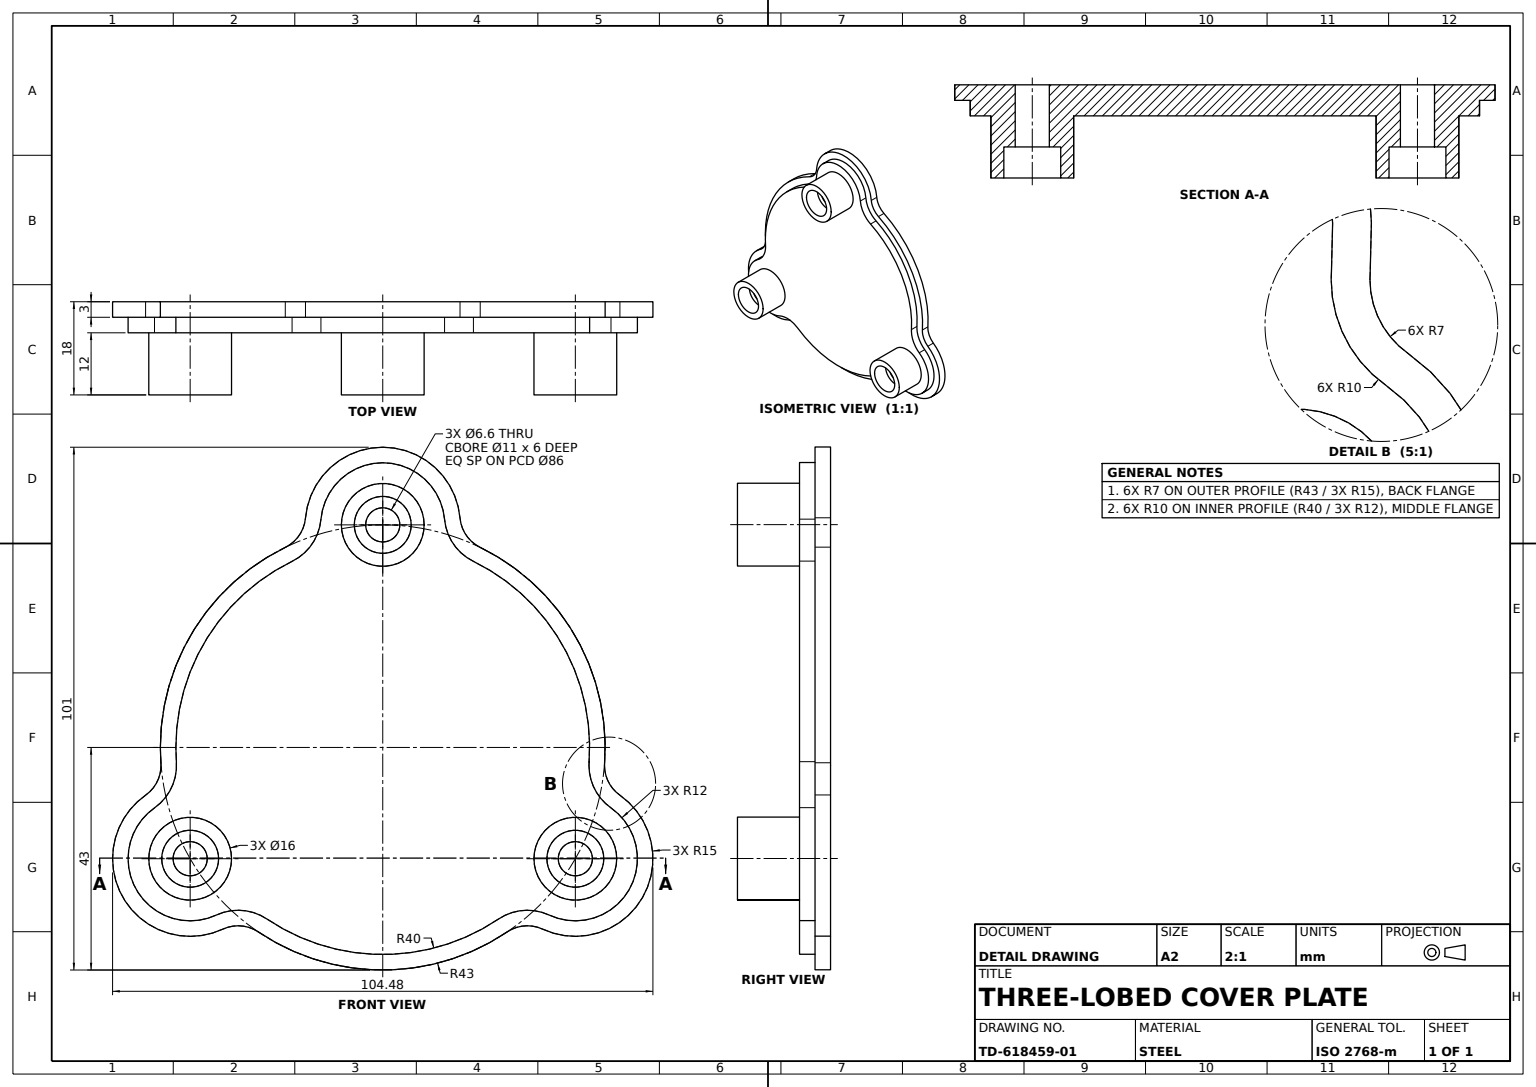
ISO-10303-21;
HEADER;
FILE_DESCRIPTION((''),'2;1');
FILE_NAME('','',(''),(''),'','','');
FILE_SCHEMA(('AUTOMOTIVE_DESIGN'));
ENDSEC;
DATA;
#1=APPLICATION_CONTEXT('');
#2=PRODUCT_CONTEXT('',#1,'mechanical');
#3=PRODUCT('','','',(#2));
#4=PRODUCT_DEFINITION_FORMATION('','',#3);
#5=PRODUCT_DEFINITION_CONTEXT('',#1,'design');
#6=PRODUCT_DEFINITION('','',#4,#5);
#7=PRODUCT_DEFINITION_SHAPE('','',#6);
#8=(LENGTH_UNIT()NAMED_UNIT(*)SI_UNIT(.MILLI.,.METRE.));
#9=(NAMED_UNIT(*)PLANE_ANGLE_UNIT()SI_UNIT($,.RADIAN.));
#10=(NAMED_UNIT(*)SI_UNIT($,.STERADIAN.)SOLID_ANGLE_UNIT());
#11=UNCERTAINTY_MEASURE_WITH_UNIT(LENGTH_MEASURE(1.E-05),#8,'distance_accuracy_value','');
#12=(GEOMETRIC_REPRESENTATION_CONTEXT(3)GLOBAL_UNCERTAINTY_ASSIGNED_CONTEXT((#11))GLOBAL_UNIT_ASSIGNED_CONTEXT((#8,#9,#10))REPRESENTATION_CONTEXT('',''));
#13=CARTESIAN_POINT('',(-31.739092,-21.5,12.));
#14=VERTEX_POINT('',#13);
#15=CARTESIAN_POINT('',(-31.739092,-21.5,18.));
#16=VERTEX_POINT('',#15);
#17=DIRECTION('',(0.,0.,1.));
#18=VECTOR('',#17,1000.);
#19=LINE('',#13,#18);
#20=EDGE_CURVE('',#14,#16,#19,.T.);
#21=ORIENTED_EDGE('',*,*,#20,.F.);
#22=CARTESIAN_POINT('',(-42.739092,-21.5,12.));
#23=VERTEX_POINT('',#22);
#24=CARTESIAN_POINT('',(-37.239092,-21.5,12.));
#25=DIRECTION('',(1.,0.,0.));
#26=AXIS2_PLACEMENT_3D('',#24,#17,#25);
#27=CIRCLE('',#26,5.5);
#28=EDGE_CURVE('',#23,#14,#27,.T.);
#29=ORIENTED_EDGE('',*,*,#28,.F.);
#30=CARTESIAN_POINT('',(-42.739092,-21.5,18.));
#31=VERTEX_POINT('',#30);
#32=LINE('',#22,#18);
#33=EDGE_CURVE('',#23,#31,#32,.T.);
#34=ORIENTED_EDGE('',*,*,#33,.T.);
#35=CARTESIAN_POINT('',(-37.239092,-21.5,18.));
#36=AXIS2_PLACEMENT_3D('',#35,#17,#25);
#37=CIRCLE('',#36,5.5);
#38=EDGE_CURVE('',#31,#16,#37,.T.);
#39=ORIENTED_EDGE('',*,*,#38,.T.);
#40=EDGE_LOOP('',(#21,#29,#34,#39));
#41=FACE_OUTER_BOUND('',#40,.T.);
#42=CYLINDRICAL_SURFACE('',#26,5.5);
#43=ADVANCED_FACE('',(#41),#42,.F.);
#44=CARTESIAN_POINT('',(-29.239092,-21.5,18.));
#45=VERTEX_POINT('',#44);
#46=CARTESIAN_POINT('',(-29.239092,-21.5,6.));
#47=VERTEX_POINT('',#46);
#48=DIRECTION('',(0.,0.,-1.));
#49=VECTOR('',#48,1000.);
#50=LINE('',#44,#49);
#51=EDGE_CURVE('',#45,#47,#50,.T.);
#52=ORIENTED_EDGE('',*,*,#51,.T.);
#53=CARTESIAN_POINT('',(-45.239092,-21.5,6.));
#54=VERTEX_POINT('',#53);
#55=CARTESIAN_POINT('',(-37.239092,-21.5,6.));
#56=AXIS2_PLACEMENT_3D('',#55,#17,#25);
#57=CIRCLE('',#56,8.);
#58=EDGE_CURVE('',#47,#54,#57,.T.);
#59=ORIENTED_EDGE('',*,*,#58,.T.);
#60=CARTESIAN_POINT('',(-45.239092,-21.5,18.));
#61=VERTEX_POINT('',#60);
#62=LINE('',#60,#49);
#63=EDGE_CURVE('',#61,#54,#62,.T.);
#64=ORIENTED_EDGE('',*,*,#63,.F.);
#65=CIRCLE('',#36,8.);
#66=EDGE_CURVE('',#45,#61,#65,.T.);
#67=ORIENTED_EDGE('',*,*,#66,.F.);
#68=EDGE_LOOP('',(#52,#59,#64,#67));
#69=FACE_OUTER_BOUND('',#68,.T.);
#70=DIRECTION('',(-1.,0.,0.));
#71=AXIS2_PLACEMENT_3D('',#35,#48,#70);
#72=CYLINDRICAL_SURFACE('',#71,8.);
#73=ADVANCED_FACE('',(#69),#72,.T.);
#74=CARTESIAN_POINT('',(-8.,43.,18.));
#75=VERTEX_POINT('',#74);
#76=CARTESIAN_POINT('',(8.,43.,18.));
#77=VERTEX_POINT('',#76);
#78=CARTESIAN_POINT('',(0.,43.,18.));
#79=AXIS2_PLACEMENT_3D('',#78,#17,#25);
#80=CIRCLE('',#79,8.);
#81=EDGE_CURVE('',#75,#77,#80,.T.);
#82=ORIENTED_EDGE('',*,*,#81,.F.);
#83=CARTESIAN_POINT('',(-8.,43.,6.));
#84=VERTEX_POINT('',#83);
#85=LINE('',#74,#49);
#86=EDGE_CURVE('',#75,#84,#85,.T.);
#87=ORIENTED_EDGE('',*,*,#86,.T.);
#88=CARTESIAN_POINT('',(8.,43.,6.));
#89=VERTEX_POINT('',#88);
#90=CARTESIAN_POINT('',(0.,43.,6.));
#91=AXIS2_PLACEMENT_3D('',#90,#17,#25);
#92=CIRCLE('',#91,8.);
#93=EDGE_CURVE('',#84,#89,#92,.T.);
#94=ORIENTED_EDGE('',*,*,#93,.T.);
#95=LINE('',#76,#49);
#96=EDGE_CURVE('',#77,#89,#95,.T.);
#97=ORIENTED_EDGE('',*,*,#96,.F.);
#98=EDGE_LOOP('',(#82,#87,#94,#97));
#99=FACE_OUTER_BOUND('',#98,.T.);
#100=AXIS2_PLACEMENT_3D('',#78,#48,#70);
#101=CYLINDRICAL_SURFACE('',#100,8.);
#102=ADVANCED_FACE('',(#99),#101,.T.);
#103=CARTESIAN_POINT('',(5.5,43.,18.));
#104=VERTEX_POINT('',#103);
#105=CARTESIAN_POINT('',(-5.5,43.,18.));
#106=VERTEX_POINT('',#105);
#107=CIRCLE('',#79,5.5);
#108=EDGE_CURVE('',#104,#106,#107,.T.);
#109=ORIENTED_EDGE('',*,*,#108,.T.);
#110=CARTESIAN_POINT('',(-5.5,43.,12.));
#111=VERTEX_POINT('',#110);
#112=LINE('',#110,#18);
#113=EDGE_CURVE('',#111,#106,#112,.T.);
#114=ORIENTED_EDGE('',*,*,#113,.F.);
#115=CARTESIAN_POINT('',(5.5,43.,12.));
#116=VERTEX_POINT('',#115);
#117=CARTESIAN_POINT('',(0.,43.,12.));
#118=AXIS2_PLACEMENT_3D('',#117,#17,#25);
#119=CIRCLE('',#118,5.5);
#120=EDGE_CURVE('',#116,#111,#119,.T.);
#121=ORIENTED_EDGE('',*,*,#120,.F.);
#122=LINE('',#115,#18);
#123=EDGE_CURVE('',#116,#104,#122,.T.);
#124=ORIENTED_EDGE('',*,*,#123,.T.);
#125=EDGE_LOOP('',(#109,#114,#121,#124));
#126=FACE_OUTER_BOUND('',#125,.T.);
#127=CYLINDRICAL_SURFACE('',#118,5.5);
#128=ADVANCED_FACE('',(#126),#127,.F.);
#129=CARTESIAN_POINT('',(-30.91498,-35.101676,3.));
#130=VERTEX_POINT('',#129);
#131=CARTESIAN_POINT('',(-24.048805,-35.646248,3.));
#132=VERTEX_POINT('',#131);
#133=CARTESIAN_POINT('',(-27.963727,-41.449125,3.));
#134=AXIS2_PLACEMENT_3D('',#133,#48,#70);
#135=CIRCLE('',#134,7.);
#136=EDGE_CURVE('',#130,#132,#135,.T.);
#137=ORIENTED_EDGE('',*,*,#136,.F.);
#138=CARTESIAN_POINT('',(-30.91498,-35.101676,0.));
#139=VERTEX_POINT('',#138);
#140=LINE('',#129,#49);
#141=EDGE_CURVE('',#130,#139,#140,.T.);
#142=ORIENTED_EDGE('',*,*,#141,.T.);
#143=CARTESIAN_POINT('',(-24.048805,-35.646248,0.));
#144=VERTEX_POINT('',#143);
#145=CARTESIAN_POINT('',(-27.963727,-41.449125,0.));
#146=AXIS2_PLACEMENT_3D('',#145,#48,#70);
#147=CIRCLE('',#146,7.);
#148=EDGE_CURVE('',#139,#144,#147,.T.);
#149=ORIENTED_EDGE('',*,*,#148,.T.);
#150=LINE('',#131,#49);
#151=EDGE_CURVE('',#132,#144,#150,.T.);
#152=ORIENTED_EDGE('',*,*,#151,.F.);
#153=EDGE_LOOP('',(#137,#142,#149,#152));
#154=FACE_OUTER_BOUND('',#153,.T.);
#155=CYLINDRICAL_SURFACE('',#134,7.);
#156=ADVANCED_FACE('',(#154),#155,.F.);
#157=CARTESIAN_POINT('',(39.877859,-3.492735,6.));
#158=VERTEX_POINT('',#157);
#159=CARTESIAN_POINT('',(39.877859,-3.492735,3.));
#160=VERTEX_POINT('',#159);
#161=LINE('',#157,#49);
#162=EDGE_CURVE('',#158,#160,#161,.T.);
#163=ORIENTED_EDGE('',*,*,#162,.F.);
#164=CARTESIAN_POINT('',(44.132965,-11.677856,6.));
#165=VERTEX_POINT('',#164);
#166=CARTESIAN_POINT('',(49.877859,-3.492735,6.));
#167=AXIS2_PLACEMENT_3D('',#166,#17,#25);
#168=CIRCLE('',#167,10.);
#169=EDGE_CURVE('',#158,#165,#168,.T.);
#170=ORIENTED_EDGE('',*,*,#169,.T.);
#171=CARTESIAN_POINT('',(44.132965,-11.677856,3.));
#172=VERTEX_POINT('',#171);
#173=LINE('',#164,#49);
#174=EDGE_CURVE('',#165,#172,#173,.T.);
#175=ORIENTED_EDGE('',*,*,#174,.T.);
#176=CARTESIAN_POINT('',(49.877859,-3.492735,3.));
#177=AXIS2_PLACEMENT_3D('',#176,#17,#25);
#178=CIRCLE('',#177,10.);
#179=EDGE_CURVE('',#160,#172,#178,.T.);
#180=ORIENTED_EDGE('',*,*,#179,.F.);
#181=EDGE_LOOP('',(#163,#170,#175,#180));
#182=FACE_OUTER_BOUND('',#181,.T.);
#183=AXIS2_PLACEMENT_3D('',#166,#48,#70);
#184=CYLINDRICAL_SURFACE('',#183,10.);
#185=ADVANCED_FACE('',(#182),#184,.F.);
#186=CARTESIAN_POINT('',(3.3,43.,0.));
#187=VERTEX_POINT('',#186);
#188=CARTESIAN_POINT('',(3.3,43.,12.));
#189=VERTEX_POINT('',#188);
#190=CARTESIAN_POINT('',(3.3,43.,-134.));
#191=LINE('',#190,#18);
#192=EDGE_CURVE('',#187,#189,#191,.T.);
#193=ORIENTED_EDGE('',*,*,#192,.F.);
#194=CARTESIAN_POINT('',(-3.3,43.,0.));
#195=VERTEX_POINT('',#194);
#196=CARTESIAN_POINT('',(0.,43.,0.));
#197=AXIS2_PLACEMENT_3D('',#196,#48,#70);
#198=CIRCLE('',#197,3.3);
#199=EDGE_CURVE('',#187,#195,#198,.T.);
#200=ORIENTED_EDGE('',*,*,#199,.T.);
#201=CARTESIAN_POINT('',(-3.3,43.,12.));
#202=VERTEX_POINT('',#201);
#203=CARTESIAN_POINT('',(-3.3,43.,-134.));
#204=LINE('',#203,#18);
#205=EDGE_CURVE('',#195,#202,#204,.T.);
#206=ORIENTED_EDGE('',*,*,#205,.T.);
#207=CIRCLE('',#118,3.3);
#208=EDGE_CURVE('',#202,#189,#207,.T.);
#209=ORIENTED_EDGE('',*,*,#208,.T.);
#210=EDGE_LOOP('',(#193,#200,#206,#209));
#211=FACE_OUTER_BOUND('',#210,.T.);
#212=CARTESIAN_POINT('',(0.,43.,-134.));
#213=AXIS2_PLACEMENT_3D('',#212,#17,#25);
#214=CYLINDRICAL_SURFACE('',#213,3.3);
#215=ADVANCED_FACE('',(#211),#214,.F.);
#216=CARTESIAN_POINT('',(45.239092,-21.5,18.));
#217=VERTEX_POINT('',#216);
#218=CARTESIAN_POINT('',(29.239092,-21.5,18.));
#219=VERTEX_POINT('',#218);
#220=CARTESIAN_POINT('',(37.239092,-21.5,18.));
#221=AXIS2_PLACEMENT_3D('',#220,#17,#25);
#222=CIRCLE('',#221,8.);
#223=EDGE_CURVE('',#217,#219,#222,.T.);
#224=ORIENTED_EDGE('',*,*,#223,.F.);
#225=CARTESIAN_POINT('',(45.239092,-21.5,6.));
#226=VERTEX_POINT('',#225);
#227=LINE('',#216,#49);
#228=EDGE_CURVE('',#217,#226,#227,.T.);
#229=ORIENTED_EDGE('',*,*,#228,.T.);
#230=CARTESIAN_POINT('',(29.239092,-21.5,6.));
#231=VERTEX_POINT('',#230);
#232=CARTESIAN_POINT('',(37.239092,-21.5,6.));
#233=AXIS2_PLACEMENT_3D('',#232,#17,#25);
#234=CIRCLE('',#233,8.);
#235=EDGE_CURVE('',#226,#231,#234,.T.);
#236=ORIENTED_EDGE('',*,*,#235,.T.);
#237=LINE('',#218,#49);
#238=EDGE_CURVE('',#219,#231,#237,.T.);
#239=ORIENTED_EDGE('',*,*,#238,.F.);
#240=EDGE_LOOP('',(#224,#229,#236,#239));
#241=FACE_OUTER_BOUND('',#240,.T.);
#242=AXIS2_PLACEMENT_3D('',#220,#48,#70);
#243=CYLINDRICAL_SURFACE('',#242,8.);
#244=ADVANCED_FACE('',(#241),#243,.T.);
#245=CARTESIAN_POINT('',(22.370982,-33.1593,6.));
#246=VERTEX_POINT('',#245);
#247=CARTESIAN_POINT('',(22.370982,-33.1593,3.));
#248=VERTEX_POINT('',#247);
#249=LINE('',#245,#49);
#250=EDGE_CURVE('',#246,#248,#249,.T.);
#251=ORIENTED_EDGE('',*,*,#250,.T.);
#252=CARTESIAN_POINT('',(32.179802,-32.381341,3.));
#253=VERTEX_POINT('',#252);
#254=CARTESIAN_POINT('',(27.963727,-41.449125,3.));
#255=AXIS2_PLACEMENT_3D('',#254,#17,#25);
#256=CIRCLE('',#255,10.);
#257=EDGE_CURVE('',#253,#248,#256,.T.);
#258=ORIENTED_EDGE('',*,*,#257,.F.);
#259=CARTESIAN_POINT('',(32.179802,-32.381341,6.));
#260=VERTEX_POINT('',#259);
#261=LINE('',#259,#49);
#262=EDGE_CURVE('',#260,#253,#261,.T.);
#263=ORIENTED_EDGE('',*,*,#262,.F.);
#264=CARTESIAN_POINT('',(27.963727,-41.449125,6.));
#265=AXIS2_PLACEMENT_3D('',#264,#17,#25);
#266=CIRCLE('',#265,10.);
#267=EDGE_CURVE('',#260,#246,#266,.T.);
#268=ORIENTED_EDGE('',*,*,#267,.T.);
#269=EDGE_LOOP('',(#251,#258,#263,#268));
#270=FACE_OUTER_BOUND('',#269,.T.);
#271=AXIS2_PLACEMENT_3D('',#264,#48,#70);
#272=CYLINDRICAL_SURFACE('',#271,10.);
#273=ADVANCED_FACE('',(#270),#272,.F.);
#274=CARTESIAN_POINT('',(-40.,0.,6.));
#275=VERTEX_POINT('',#274);
#276=CARTESIAN_POINT('',(-40.,0.,3.));
#277=VERTEX_POINT('',#276);
#278=LINE('',#274,#49);
#279=EDGE_CURVE('',#275,#277,#278,.T.);
#280=ORIENTED_EDGE('',*,*,#279,.F.);
#281=CARTESIAN_POINT('',(-17.531306,35.953488,6.));
#282=VERTEX_POINT('',#281);
#283=CARTESIAN_POINT('',(0.,0.,6.));
#284=AXIS2_PLACEMENT_3D('',#283,#17,#25);
#285=CIRCLE('',#284,40.);
#286=EDGE_CURVE('',#282,#275,#285,.T.);
#287=ORIENTED_EDGE('',*,*,#286,.F.);
#288=CARTESIAN_POINT('',(-17.531306,35.953488,3.));
#289=VERTEX_POINT('',#288);
#290=LINE('',#281,#49);
#291=EDGE_CURVE('',#282,#289,#290,.T.);
#292=ORIENTED_EDGE('',*,*,#291,.T.);
#293=CARTESIAN_POINT('',(0.,0.,3.));
#294=AXIS2_PLACEMENT_3D('',#293,#17,#25);
#295=CIRCLE('',#294,40.);
#296=EDGE_CURVE('',#289,#277,#295,.T.);
#297=ORIENTED_EDGE('',*,*,#296,.T.);
#298=EDGE_LOOP('',(#280,#287,#292,#297));
#299=FACE_OUTER_BOUND('',#298,.T.);
#300=AXIS2_PLACEMENT_3D('',#283,#48,#70);
#301=CYLINDRICAL_SURFACE('',#300,40.);
#302=ADVANCED_FACE('',(#299),#301,.T.);
#303=CARTESIAN_POINT('',(40.539092,-21.5,12.));
#304=VERTEX_POINT('',#303);
#305=CARTESIAN_POINT('',(33.939092,-21.5,12.));
#306=VERTEX_POINT('',#305);
#307=CARTESIAN_POINT('',(37.239092,-21.5,12.));
#308=AXIS2_PLACEMENT_3D('',#307,#17,#25);
#309=CIRCLE('',#308,3.3);
#310=EDGE_CURVE('',#304,#306,#309,.T.);
#311=ORIENTED_EDGE('',*,*,#310,.F.);
#312=EDGE_CURVE('',#306,#304,#309,.T.);
#313=ORIENTED_EDGE('',*,*,#312,.F.);
#314=EDGE_LOOP('',(#311,#313));
#315=FACE_BOUND('',#314,.T.);
#316=CARTESIAN_POINT('',(31.739092,-21.5,12.));
#317=VERTEX_POINT('',#316);
#318=CARTESIAN_POINT('',(42.739092,-21.5,12.));
#319=VERTEX_POINT('',#318);
#320=CIRCLE('',#308,5.5);
#321=EDGE_CURVE('',#317,#319,#320,.T.);
#322=ORIENTED_EDGE('',*,*,#321,.T.);
#323=EDGE_CURVE('',#319,#317,#320,.T.);
#324=ORIENTED_EDGE('',*,*,#323,.T.);
#325=EDGE_LOOP('',(#322,#324));
#326=FACE_OUTER_BOUND('',#325,.T.);
#327=PLANE('',#308);
#328=ADVANCED_FACE('',(#315,#326),#327,.T.);
#329=CARTESIAN_POINT('',(11.953163,44.059197,6.));
#330=VERTEX_POINT('',#329);
#331=CARTESIAN_POINT('',(-11.953163,44.059197,6.));
#332=VERTEX_POINT('',#331);
#333=CIRCLE('',#91,12.);
#334=EDGE_CURVE('',#330,#332,#333,.T.);
#335=ORIENTED_EDGE('',*,*,#334,.F.);
#336=CARTESIAN_POINT('',(11.953163,44.059197,3.));
#337=VERTEX_POINT('',#336);
#338=LINE('',#329,#49);
#339=EDGE_CURVE('',#330,#337,#338,.T.);
#340=ORIENTED_EDGE('',*,*,#339,.T.);
#341=CARTESIAN_POINT('',(-11.953163,44.059197,3.));
#342=VERTEX_POINT('',#341);
#343=CARTESIAN_POINT('',(0.,43.,3.));
#344=AXIS2_PLACEMENT_3D('',#343,#17,#25);
#345=CIRCLE('',#344,12.);
#346=EDGE_CURVE('',#337,#342,#345,.T.);
#347=ORIENTED_EDGE('',*,*,#346,.T.);
#348=LINE('',#331,#49);
#349=EDGE_CURVE('',#332,#342,#348,.T.);
#350=ORIENTED_EDGE('',*,*,#349,.F.);
#351=EDGE_LOOP('',(#335,#340,#347,#350));
#352=FACE_OUTER_BOUND('',#351,.T.);
#353=AXIS2_PLACEMENT_3D('',#90,#48,#70);
#354=CYLINDRICAL_SURFACE('',#353,12.);
#355=ADVANCED_FACE('',(#352),#354,.T.);
#356=CARTESIAN_POINT('',(-49.239092,-21.5,6.));
#357=VERTEX_POINT('',#356);
#358=CARTESIAN_POINT('',(-49.239092,-21.5,3.));
#359=VERTEX_POINT('',#358);
#360=LINE('',#356,#49);
#361=EDGE_CURVE('',#357,#359,#360,.T.);
#362=ORIENTED_EDGE('',*,*,#361,.T.);
#363=CARTESIAN_POINT('',(-32.179802,-32.381341,3.));
#364=VERTEX_POINT('',#363);
#365=CARTESIAN_POINT('',(-37.239092,-21.5,3.));
#366=AXIS2_PLACEMENT_3D('',#365,#17,#25);
#367=CIRCLE('',#366,12.);
#368=EDGE_CURVE('',#359,#364,#367,.T.);
#369=ORIENTED_EDGE('',*,*,#368,.T.);
#370=CARTESIAN_POINT('',(-32.179802,-32.381341,6.));
#371=VERTEX_POINT('',#370);
#372=LINE('',#370,#49);
#373=EDGE_CURVE('',#371,#364,#372,.T.);
#374=ORIENTED_EDGE('',*,*,#373,.F.);
#375=CIRCLE('',#56,12.);
#376=EDGE_CURVE('',#357,#371,#375,.T.);
#377=ORIENTED_EDGE('',*,*,#376,.F.);
#378=EDGE_LOOP('',(#362,#369,#374,#377));
#379=FACE_OUTER_BOUND('',#378,.T.);
#380=AXIS2_PLACEMENT_3D('',#55,#48,#70);
#381=CYLINDRICAL_SURFACE('',#380,12.);
#382=ADVANCED_FACE('',(#379),#381,.T.);
#383=CARTESIAN_POINT('',(-39.902287,-2.794188,6.));
#384=VERTEX_POINT('',#383);
#385=CARTESIAN_POINT('',(-39.902287,-2.794188,3.));
#386=VERTEX_POINT('',#385);
#387=LINE('',#383,#49);
#388=EDGE_CURVE('',#384,#386,#387,.T.);
#389=ORIENTED_EDGE('',*,*,#388,.T.);
#390=CARTESIAN_POINT('',(-44.132965,-11.677856,3.));
#391=VERTEX_POINT('',#390);
#392=CARTESIAN_POINT('',(-49.877859,-3.492735,3.));
#393=AXIS2_PLACEMENT_3D('',#392,#17,#25);
#394=CIRCLE('',#393,10.);
#395=EDGE_CURVE('',#391,#386,#394,.T.);
#396=ORIENTED_EDGE('',*,*,#395,.F.);
#397=CARTESIAN_POINT('',(-44.132965,-11.677856,6.));
#398=VERTEX_POINT('',#397);
#399=LINE('',#397,#49);
#400=EDGE_CURVE('',#398,#391,#399,.T.);
#401=ORIENTED_EDGE('',*,*,#400,.F.);
#402=CARTESIAN_POINT('',(-49.877859,-3.492735,6.));
#403=AXIS2_PLACEMENT_3D('',#402,#17,#25);
#404=CIRCLE('',#403,10.);
#405=EDGE_CURVE('',#398,#384,#404,.T.);
#406=ORIENTED_EDGE('',*,*,#405,.T.);
#407=EDGE_LOOP('',(#389,#396,#401,#406));
#408=FACE_OUTER_BOUND('',#407,.T.);
#409=AXIS2_PLACEMENT_3D('',#402,#48,#70);
#410=CYLINDRICAL_SURFACE('',#409,10.);
#411=ADVANCED_FACE('',(#408),#410,.F.);
#412=CARTESIAN_POINT('',(-42.894959,-3.003752,0.));
#413=VERTEX_POINT('',#412);
#414=CARTESIAN_POINT('',(-45.856433,-9.22232,0.));
#415=VERTEX_POINT('',#414);
#416=CARTESIAN_POINT('',(-49.877859,-3.492735,0.));
#417=AXIS2_PLACEMENT_3D('',#416,#48,#25);
#418=CIRCLE('',#417,7.);
#419=EDGE_CURVE('',#413,#415,#418,.T.);
#420=ORIENTED_EDGE('',*,*,#419,.T.);
#421=CARTESIAN_POINT('',(-45.856433,-9.22232,3.));
#422=VERTEX_POINT('',#421);
#423=LINE('',#421,#49);
#424=EDGE_CURVE('',#422,#415,#423,.T.);
#425=ORIENTED_EDGE('',*,*,#424,.F.);
#426=CARTESIAN_POINT('',(-42.894959,-3.003752,3.));
#427=VERTEX_POINT('',#426);
#428=AXIS2_PLACEMENT_3D('',#392,#48,#25);
#429=CIRCLE('',#428,7.);
#430=EDGE_CURVE('',#427,#422,#429,.T.);
#431=ORIENTED_EDGE('',*,*,#430,.F.);
#432=LINE('',#426,#49);
#433=EDGE_CURVE('',#427,#413,#432,.T.);
#434=ORIENTED_EDGE('',*,*,#433,.T.);
#435=EDGE_LOOP('',(#420,#425,#431,#434));
#436=FACE_OUTER_BOUND('',#435,.T.);
#437=AXIS2_PLACEMENT_3D('',#392,#48,#70);
#438=CYLINDRICAL_SURFACE('',#437,7.);
#439=ADVANCED_FACE('',(#436),#438,.F.);
#440=EDGE_CURVE('',#14,#23,#27,.T.);
#441=ORIENTED_EDGE('',*,*,#440,.T.);
#442=ORIENTED_EDGE('',*,*,#28,.T.);
#443=EDGE_LOOP('',(#441,#442));
#444=FACE_OUTER_BOUND('',#443,.T.);
#445=CARTESIAN_POINT('',(-40.539092,-21.5,12.));
#446=VERTEX_POINT('',#445);
#447=CARTESIAN_POINT('',(-33.939092,-21.5,12.));
#448=VERTEX_POINT('',#447);
#449=CIRCLE('',#26,3.3);
#450=EDGE_CURVE('',#446,#448,#449,.T.);
#451=ORIENTED_EDGE('',*,*,#450,.F.);
#452=EDGE_CURVE('',#448,#446,#449,.T.);
#453=ORIENTED_EDGE('',*,*,#452,.F.);
#454=EDGE_LOOP('',(#451,#453));
#455=FACE_BOUND('',#454,.T.);
#456=PLANE('',#26);
#457=ADVANCED_FACE('',(#444,#455),#456,.T.);
#458=CARTESIAN_POINT('',(-14.941454,44.323996,3.));
#459=VERTEX_POINT('',#458);
#460=CARTESIAN_POINT('',(-18.846153,38.65,3.));
#461=VERTEX_POINT('',#460);
#462=CARTESIAN_POINT('',(-21.914132,44.94186,3.));
#463=AXIS2_PLACEMENT_3D('',#462,#48,#70);
#464=CIRCLE('',#463,7.);
#465=EDGE_CURVE('',#459,#461,#464,.T.);
#466=ORIENTED_EDGE('',*,*,#465,.F.);
#467=CARTESIAN_POINT('',(-14.941454,44.323996,0.));
#468=VERTEX_POINT('',#467);
#469=LINE('',#458,#49);
#470=EDGE_CURVE('',#459,#468,#469,.T.);
#471=ORIENTED_EDGE('',*,*,#470,.T.);
#472=CARTESIAN_POINT('',(-18.846153,38.65,0.));
#473=VERTEX_POINT('',#472);
#474=CARTESIAN_POINT('',(-21.914132,44.94186,0.));
#475=AXIS2_PLACEMENT_3D('',#474,#48,#70);
#476=CIRCLE('',#475,7.);
#477=EDGE_CURVE('',#468,#473,#476,.T.);
#478=ORIENTED_EDGE('',*,*,#477,.T.);
#479=LINE('',#460,#49);
#480=EDGE_CURVE('',#461,#473,#479,.T.);
#481=ORIENTED_EDGE('',*,*,#480,.F.);
#482=EDGE_LOOP('',(#466,#471,#478,#481));
#483=FACE_OUTER_BOUND('',#482,.T.);
#484=CYLINDRICAL_SURFACE('',#463,7.);
#485=ADVANCED_FACE('',(#483),#484,.F.);
#486=CARTESIAN_POINT('',(-33.939092,-21.5,0.));
#487=VERTEX_POINT('',#486);
#488=CARTESIAN_POINT('',(-33.939092,-21.5,-134.));
#489=LINE('',#488,#18);
#490=EDGE_CURVE('',#487,#448,#489,.T.);
#491=ORIENTED_EDGE('',*,*,#490,.F.);
#492=CARTESIAN_POINT('',(-40.539092,-21.5,0.));
#493=VERTEX_POINT('',#492);
#494=CARTESIAN_POINT('',(-37.239092,-21.5,0.));
#495=AXIS2_PLACEMENT_3D('',#494,#48,#70);
#496=CIRCLE('',#495,3.3);
#497=EDGE_CURVE('',#487,#493,#496,.T.);
#498=ORIENTED_EDGE('',*,*,#497,.T.);
#499=CARTESIAN_POINT('',(-40.539092,-21.5,-134.));
#500=LINE('',#499,#18);
#501=EDGE_CURVE('',#493,#446,#500,.T.);
#502=ORIENTED_EDGE('',*,*,#501,.T.);
#503=ORIENTED_EDGE('',*,*,#450,.T.);
#504=EDGE_LOOP('',(#491,#498,#502,#503));
#505=FACE_OUTER_BOUND('',#504,.T.);
#506=CARTESIAN_POINT('',(-37.239092,-21.5,-134.));
#507=AXIS2_PLACEMENT_3D('',#506,#17,#25);
#508=CYLINDRICAL_SURFACE('',#507,3.3);
#509=ADVANCED_FACE('',(#505),#508,.F.);
#510=CARTESIAN_POINT('',(-21.914132,44.94186,6.));
#511=AXIS2_PLACEMENT_3D('',#510,#17,#25);
#512=CIRCLE('',#511,10.);
#513=EDGE_CURVE('',#282,#332,#512,.T.);
#514=ORIENTED_EDGE('',*,*,#513,.T.);
#515=ORIENTED_EDGE('',*,*,#349,.T.);
#516=AXIS2_PLACEMENT_3D('',#462,#17,#25);
#517=CIRCLE('',#516,10.);
#518=EDGE_CURVE('',#289,#342,#517,.T.);
#519=ORIENTED_EDGE('',*,*,#518,.F.);
#520=ORIENTED_EDGE('',*,*,#291,.F.);
#521=EDGE_LOOP('',(#514,#515,#519,#520));
#522=FACE_OUTER_BOUND('',#521,.T.);
#523=AXIS2_PLACEMENT_3D('',#510,#48,#70);
#524=CYLINDRICAL_SURFACE('',#523,10.);
#525=ADVANCED_FACE('',(#522),#524,.F.);
#526=ORIENTED_EDGE('',*,*,#123,.F.);
#527=EDGE_CURVE('',#111,#116,#119,.T.);
#528=ORIENTED_EDGE('',*,*,#527,.F.);
#529=ORIENTED_EDGE('',*,*,#113,.T.);
#530=EDGE_CURVE('',#106,#104,#107,.T.);
#531=ORIENTED_EDGE('',*,*,#530,.T.);
#532=EDGE_LOOP('',(#526,#528,#529,#531));
#533=FACE_OUTER_BOUND('',#532,.T.);
#534=ADVANCED_FACE('',(#533),#127,.F.);
#535=CARTESIAN_POINT('',(31.739092,-21.5,18.));
#536=VERTEX_POINT('',#535);
#537=LINE('',#316,#18);
#538=EDGE_CURVE('',#317,#536,#537,.T.);
#539=ORIENTED_EDGE('',*,*,#538,.T.);
#540=CARTESIAN_POINT('',(42.739092,-21.5,18.));
#541=VERTEX_POINT('',#540);
#542=CIRCLE('',#221,5.5);
#543=EDGE_CURVE('',#536,#541,#542,.T.);
#544=ORIENTED_EDGE('',*,*,#543,.T.);
#545=LINE('',#318,#18);
#546=EDGE_CURVE('',#319,#541,#545,.T.);
#547=ORIENTED_EDGE('',*,*,#546,.F.);
#548=ORIENTED_EDGE('',*,*,#321,.F.);
#549=EDGE_LOOP('',(#539,#544,#547,#548));
#550=FACE_OUTER_BOUND('',#549,.T.);
#551=CYLINDRICAL_SURFACE('',#308,5.5);
#552=ADVANCED_FACE('',(#550),#551,.F.);
#553=CARTESIAN_POINT('',(33.939092,-21.5,0.));
#554=VERTEX_POINT('',#553);
#555=CARTESIAN_POINT('',(40.539092,-21.5,0.));
#556=VERTEX_POINT('',#555);
#557=CARTESIAN_POINT('',(37.239092,-21.5,0.));
#558=AXIS2_PLACEMENT_3D('',#557,#48,#70);
#559=CIRCLE('',#558,3.3);
#560=EDGE_CURVE('',#554,#556,#559,.T.);
#561=ORIENTED_EDGE('',*,*,#560,.T.);
#562=CARTESIAN_POINT('',(40.539092,-21.5,-134.));
#563=LINE('',#562,#18);
#564=EDGE_CURVE('',#556,#304,#563,.T.);
#565=ORIENTED_EDGE('',*,*,#564,.T.);
#566=ORIENTED_EDGE('',*,*,#310,.T.);
#567=CARTESIAN_POINT('',(33.939092,-21.5,-134.));
#568=LINE('',#567,#18);
#569=EDGE_CURVE('',#554,#306,#568,.T.);
#570=ORIENTED_EDGE('',*,*,#569,.F.);
#571=EDGE_LOOP('',(#561,#565,#566,#570));
#572=FACE_OUTER_BOUND('',#571,.T.);
#573=CARTESIAN_POINT('',(37.239092,-21.5,-134.));
#574=AXIS2_PLACEMENT_3D('',#573,#17,#25);
#575=CYLINDRICAL_SURFACE('',#574,3.3);
#576=ADVANCED_FACE('',(#572),#575,.F.);
#577=CARTESIAN_POINT('',(45.856433,-9.22232,3.));
#578=VERTEX_POINT('',#577);
#579=CARTESIAN_POINT('',(42.877859,-3.492735,3.));
#580=VERTEX_POINT('',#579);
#581=AXIS2_PLACEMENT_3D('',#176,#48,#70);
#582=CIRCLE('',#581,7.);
#583=EDGE_CURVE('',#578,#580,#582,.T.);
#584=ORIENTED_EDGE('',*,*,#583,.F.);
#585=CARTESIAN_POINT('',(45.856433,-9.22232,0.));
#586=VERTEX_POINT('',#585);
#587=LINE('',#577,#49);
#588=EDGE_CURVE('',#578,#586,#587,.T.);
#589=ORIENTED_EDGE('',*,*,#588,.T.);
#590=CARTESIAN_POINT('',(42.877859,-3.492735,0.));
#591=VERTEX_POINT('',#590);
#592=CARTESIAN_POINT('',(49.877859,-3.492735,0.));
#593=AXIS2_PLACEMENT_3D('',#592,#48,#70);
#594=CIRCLE('',#593,7.);
#595=EDGE_CURVE('',#586,#591,#594,.T.);
#596=ORIENTED_EDGE('',*,*,#595,.T.);
#597=LINE('',#579,#49);
#598=EDGE_CURVE('',#580,#591,#597,.T.);
#599=ORIENTED_EDGE('',*,*,#598,.F.);
#600=EDGE_LOOP('',(#584,#589,#596,#599));
#601=FACE_OUTER_BOUND('',#600,.T.);
#602=CYLINDRICAL_SURFACE('',#581,7.);
#603=ADVANCED_FACE('',(#601),#602,.F.);
#604=CARTESIAN_POINT('',(24.048805,-35.646248,3.));
#605=VERTEX_POINT('',#604);
#606=CARTESIAN_POINT('',(24.048805,-35.646248,0.));
#607=VERTEX_POINT('',#606);
#608=LINE('',#604,#49);
#609=EDGE_CURVE('',#605,#607,#608,.T.);
#610=ORIENTED_EDGE('',*,*,#609,.T.);
#611=CARTESIAN_POINT('',(30.91498,-35.101676,0.));
#612=VERTEX_POINT('',#611);
#613=CARTESIAN_POINT('',(27.963727,-41.449125,0.));
#614=AXIS2_PLACEMENT_3D('',#613,#48,#25);
#615=CIRCLE('',#614,7.);
#616=EDGE_CURVE('',#607,#612,#615,.T.);
#617=ORIENTED_EDGE('',*,*,#616,.T.);
#618=CARTESIAN_POINT('',(30.91498,-35.101676,3.));
#619=VERTEX_POINT('',#618);
#620=LINE('',#618,#49);
#621=EDGE_CURVE('',#619,#612,#620,.T.);
#622=ORIENTED_EDGE('',*,*,#621,.F.);
#623=AXIS2_PLACEMENT_3D('',#254,#48,#25);
#624=CIRCLE('',#623,7.);
#625=EDGE_CURVE('',#605,#619,#624,.T.);
#626=ORIENTED_EDGE('',*,*,#625,.F.);
#627=EDGE_LOOP('',(#610,#617,#622,#626));
#628=FACE_OUTER_BOUND('',#627,.T.);
#629=AXIS2_PLACEMENT_3D('',#254,#48,#70);
#630=CYLINDRICAL_SURFACE('',#629,7.);
#631=ADVANCED_FACE('',(#628),#630,.F.);
#632=CARTESIAN_POINT('',(-22.370982,-33.1593,6.));
#633=VERTEX_POINT('',#632);
#634=CARTESIAN_POINT('',(-27.963727,-41.449125,6.));
#635=AXIS2_PLACEMENT_3D('',#634,#17,#25);
#636=CIRCLE('',#635,10.);
#637=EDGE_CURVE('',#633,#371,#636,.T.);
#638=ORIENTED_EDGE('',*,*,#637,.F.);
#639=EDGE_CURVE('',#633,#246,#285,.T.);
#640=ORIENTED_EDGE('',*,*,#639,.T.);
#641=ORIENTED_EDGE('',*,*,#267,.F.);
#642=CIRCLE('',#233,12.);
#643=EDGE_CURVE('',#260,#165,#642,.T.);
#644=ORIENTED_EDGE('',*,*,#643,.T.);
#645=ORIENTED_EDGE('',*,*,#169,.F.);
#646=CARTESIAN_POINT('',(39.902287,-2.794188,6.));
#647=VERTEX_POINT('',#646);
#648=EDGE_CURVE('',#647,#158,#168,.T.);
#649=ORIENTED_EDGE('',*,*,#648,.F.);
#650=CARTESIAN_POINT('',(17.531306,35.953488,6.));
#651=VERTEX_POINT('',#650);
#652=EDGE_CURVE('',#647,#651,#285,.T.);
#653=ORIENTED_EDGE('',*,*,#652,.T.);
#654=CARTESIAN_POINT('',(21.914132,44.94186,6.));
#655=AXIS2_PLACEMENT_3D('',#654,#17,#25);
#656=CIRCLE('',#655,10.);
#657=EDGE_CURVE('',#330,#651,#656,.T.);
#658=ORIENTED_EDGE('',*,*,#657,.F.);
#659=ORIENTED_EDGE('',*,*,#334,.T.);
#660=ORIENTED_EDGE('',*,*,#513,.F.);
#661=ORIENTED_EDGE('',*,*,#286,.T.);
#662=EDGE_CURVE('',#275,#384,#285,.T.);
#663=ORIENTED_EDGE('',*,*,#662,.T.);
#664=ORIENTED_EDGE('',*,*,#405,.F.);
#665=EDGE_CURVE('',#398,#357,#375,.T.);
#666=ORIENTED_EDGE('',*,*,#665,.T.);
#667=ORIENTED_EDGE('',*,*,#376,.T.);
#668=EDGE_LOOP('',(#638,#640,#641,#644,#645,#649,#653,#658,#659,#660,#661,#663,#664,#666,#667));
#669=FACE_OUTER_BOUND('',#668,.T.);
#670=EDGE_CURVE('',#54,#47,#57,.T.);
#671=ORIENTED_EDGE('',*,*,#670,.F.);
#672=ORIENTED_EDGE('',*,*,#58,.F.);
#673=EDGE_LOOP('',(#671,#672));
#674=FACE_BOUND('',#673,.T.);
#675=ORIENTED_EDGE('',*,*,#235,.F.);
#676=EDGE_CURVE('',#231,#226,#234,.T.);
#677=ORIENTED_EDGE('',*,*,#676,.F.);
#678=EDGE_LOOP('',(#675,#677));
#679=FACE_BOUND('',#678,.T.);
#680=ORIENTED_EDGE('',*,*,#93,.F.);
#681=EDGE_CURVE('',#89,#84,#92,.T.);
#682=ORIENTED_EDGE('',*,*,#681,.F.);
#683=EDGE_LOOP('',(#680,#682));
#684=FACE_BOUND('',#683,.T.);
#685=PLANE('',#284);
#686=ADVANCED_FACE('',(#669,#674,#679,#684),#685,.T.);
#687=ORIENTED_EDGE('',*,*,#470,.F.);
#688=CARTESIAN_POINT('',(14.941454,44.323996,3.));
#689=VERTEX_POINT('',#688);
#690=CIRCLE('',#344,15.);
#691=EDGE_CURVE('',#689,#459,#690,.T.);
#692=ORIENTED_EDGE('',*,*,#691,.F.);
#693=CARTESIAN_POINT('',(14.941454,44.323996,0.));
#694=VERTEX_POINT('',#693);
#695=LINE('',#688,#49);
#696=EDGE_CURVE('',#689,#694,#695,.T.);
#697=ORIENTED_EDGE('',*,*,#696,.T.);
#698=AXIS2_PLACEMENT_3D('',#196,#17,#25);
#699=CIRCLE('',#698,15.);
#700=EDGE_CURVE('',#694,#468,#699,.T.);
#701=ORIENTED_EDGE('',*,*,#700,.T.);
#702=EDGE_LOOP('',(#687,#692,#697,#701));
#703=FACE_OUTER_BOUND('',#702,.T.);
#704=AXIS2_PLACEMENT_3D('',#343,#48,#70);
#705=CYLINDRICAL_SURFACE('',#704,15.);
#706=ADVANCED_FACE('',(#703),#705,.T.);
#707=CIRCLE('',#294,43.);
#708=EDGE_CURVE('',#132,#605,#707,.T.);
#709=ORIENTED_EDGE('',*,*,#708,.F.);
#710=ORIENTED_EDGE('',*,*,#151,.T.);
#711=CARTESIAN_POINT('',(0.,0.,0.));
#712=AXIS2_PLACEMENT_3D('',#711,#17,#25);
#713=CIRCLE('',#712,43.);
#714=EDGE_CURVE('',#144,#607,#713,.T.);
#715=ORIENTED_EDGE('',*,*,#714,.T.);
#716=ORIENTED_EDGE('',*,*,#609,.F.);
#717=EDGE_LOOP('',(#709,#710,#715,#716));
#718=FACE_OUTER_BOUND('',#717,.T.);
#719=AXIS2_PLACEMENT_3D('',#293,#48,#70);
#720=CYLINDRICAL_SURFACE('',#719,43.);
#721=ADVANCED_FACE('',(#718),#720,.T.);
#722=CARTESIAN_POINT('',(-43.,0.,0.));
#723=VERTEX_POINT('',#722);
#724=EDGE_CURVE('',#473,#723,#713,.T.);
#725=ORIENTED_EDGE('',*,*,#724,.T.);
#726=CARTESIAN_POINT('',(-43.,0.,3.));
#727=VERTEX_POINT('',#726);
#728=LINE('',#726,#49);
#729=EDGE_CURVE('',#727,#723,#728,.T.);
#730=ORIENTED_EDGE('',*,*,#729,.F.);
#731=EDGE_CURVE('',#461,#727,#707,.T.);
#732=ORIENTED_EDGE('',*,*,#731,.F.);
#733=ORIENTED_EDGE('',*,*,#480,.T.);
#734=EDGE_LOOP('',(#725,#730,#732,#733));
#735=FACE_OUTER_BOUND('',#734,.T.);
#736=ADVANCED_FACE('',(#735),#720,.T.);
#737=ORIENTED_EDGE('',*,*,#424,.T.);
#738=CARTESIAN_POINT('',(-52.239092,-21.5,0.));
#739=VERTEX_POINT('',#738);
#740=AXIS2_PLACEMENT_3D('',#494,#17,#25);
#741=CIRCLE('',#740,15.);
#742=EDGE_CURVE('',#415,#739,#741,.T.);
#743=ORIENTED_EDGE('',*,*,#742,.T.);
#744=CARTESIAN_POINT('',(-52.239092,-21.5,3.));
#745=VERTEX_POINT('',#744);
#746=LINE('',#744,#49);
#747=EDGE_CURVE('',#745,#739,#746,.T.);
#748=ORIENTED_EDGE('',*,*,#747,.F.);
#749=CIRCLE('',#366,15.);
#750=EDGE_CURVE('',#422,#745,#749,.T.);
#751=ORIENTED_EDGE('',*,*,#750,.F.);
#752=EDGE_LOOP('',(#737,#743,#748,#751));
#753=FACE_OUTER_BOUND('',#752,.T.);
#754=AXIS2_PLACEMENT_3D('',#365,#48,#70);
#755=CYLINDRICAL_SURFACE('',#754,15.);
#756=ADVANCED_FACE('',(#753),#755,.T.);
#757=EDGE_CURVE('',#195,#187,#198,.T.);
#758=ORIENTED_EDGE('',*,*,#757,.T.);
#759=ORIENTED_EDGE('',*,*,#192,.T.);
#760=EDGE_CURVE('',#189,#202,#207,.T.);
#761=ORIENTED_EDGE('',*,*,#760,.T.);
#762=ORIENTED_EDGE('',*,*,#205,.F.);
#763=EDGE_LOOP('',(#758,#759,#761,#762));
#764=FACE_OUTER_BOUND('',#763,.T.);
#765=ADVANCED_FACE('',(#764),#214,.F.);
#766=ORIENTED_EDGE('',*,*,#81,.T.);
#767=EDGE_CURVE('',#77,#75,#80,.T.);
#768=ORIENTED_EDGE('',*,*,#767,.T.);
#769=EDGE_LOOP('',(#766,#768));
#770=FACE_OUTER_BOUND('',#769,.T.);
#771=ORIENTED_EDGE('',*,*,#108,.F.);
#772=ORIENTED_EDGE('',*,*,#530,.F.);
#773=EDGE_LOOP('',(#771,#772));
#774=FACE_BOUND('',#773,.T.);
#775=PLANE('',#79);
#776=ADVANCED_FACE('',(#770,#774),#775,.T.);
#777=CARTESIAN_POINT('',(-22.370982,-33.1593,3.));
#778=VERTEX_POINT('',#777);
#779=LINE('',#632,#49);
#780=EDGE_CURVE('',#633,#778,#779,.T.);
#781=ORIENTED_EDGE('',*,*,#780,.F.);
#782=ORIENTED_EDGE('',*,*,#637,.T.);
#783=ORIENTED_EDGE('',*,*,#373,.T.);
#784=AXIS2_PLACEMENT_3D('',#133,#17,#25);
#785=CIRCLE('',#784,10.);
#786=EDGE_CURVE('',#778,#364,#785,.T.);
#787=ORIENTED_EDGE('',*,*,#786,.F.);
#788=EDGE_LOOP('',(#781,#782,#783,#787));
#789=FACE_OUTER_BOUND('',#788,.T.);
#790=AXIS2_PLACEMENT_3D('',#634,#48,#70);
#791=CYLINDRICAL_SURFACE('',#790,10.);
#792=ADVANCED_FACE('',(#789),#791,.F.);
#793=ORIENTED_EDGE('',*,*,#120,.T.);
#794=ORIENTED_EDGE('',*,*,#527,.T.);
#795=EDGE_LOOP('',(#793,#794));
#796=FACE_OUTER_BOUND('',#795,.T.);
#797=ORIENTED_EDGE('',*,*,#208,.F.);
#798=ORIENTED_EDGE('',*,*,#760,.F.);
#799=EDGE_LOOP('',(#797,#798));
#800=FACE_BOUND('',#799,.T.);
#801=PLANE('',#118);
#802=ADVANCED_FACE('',(#796,#800),#801,.T.);
#803=ORIENTED_EDGE('',*,*,#621,.T.);
#804=AXIS2_PLACEMENT_3D('',#557,#17,#25);
#805=CIRCLE('',#804,15.);
#806=EDGE_CURVE('',#612,#586,#805,.T.);
#807=ORIENTED_EDGE('',*,*,#806,.T.);
#808=ORIENTED_EDGE('',*,*,#588,.F.);
#809=CARTESIAN_POINT('',(37.239092,-21.5,3.));
#810=AXIS2_PLACEMENT_3D('',#809,#17,#25);
#811=CIRCLE('',#810,15.);
#812=EDGE_CURVE('',#619,#578,#811,.T.);
#813=ORIENTED_EDGE('',*,*,#812,.F.);
#814=EDGE_LOOP('',(#803,#807,#808,#813));
#815=FACE_OUTER_BOUND('',#814,.T.);
#816=AXIS2_PLACEMENT_3D('',#809,#48,#70);
#817=CYLINDRICAL_SURFACE('',#816,15.);
#818=ADVANCED_FACE('',(#815),#817,.T.);
#819=ORIENTED_EDGE('',*,*,#676,.T.);
#820=ORIENTED_EDGE('',*,*,#228,.F.);
#821=EDGE_CURVE('',#219,#217,#222,.T.);
#822=ORIENTED_EDGE('',*,*,#821,.F.);
#823=ORIENTED_EDGE('',*,*,#238,.T.);
#824=EDGE_LOOP('',(#819,#820,#822,#823));
#825=FACE_OUTER_BOUND('',#824,.T.);
#826=ADVANCED_FACE('',(#825),#243,.T.);
#827=ORIENTED_EDGE('',*,*,#339,.F.);
#828=ORIENTED_EDGE('',*,*,#657,.T.);
#829=CARTESIAN_POINT('',(17.531306,35.953488,3.));
#830=VERTEX_POINT('',#829);
#831=LINE('',#650,#49);
#832=EDGE_CURVE('',#651,#830,#831,.T.);
#833=ORIENTED_EDGE('',*,*,#832,.T.);
#834=CARTESIAN_POINT('',(21.914132,44.94186,3.));
#835=AXIS2_PLACEMENT_3D('',#834,#17,#25);
#836=CIRCLE('',#835,10.);
#837=EDGE_CURVE('',#337,#830,#836,.T.);
#838=ORIENTED_EDGE('',*,*,#837,.F.);
#839=EDGE_LOOP('',(#827,#828,#833,#838));
#840=FACE_OUTER_BOUND('',#839,.T.);
#841=AXIS2_PLACEMENT_3D('',#654,#48,#70);
#842=CYLINDRICAL_SURFACE('',#841,10.);
#843=ADVANCED_FACE('',(#840),#842,.F.);
#844=CARTESIAN_POINT('',(18.846153,38.65,3.));
#845=VERTEX_POINT('',#844);
#846=CARTESIAN_POINT('',(18.846153,38.65,0.));
#847=VERTEX_POINT('',#846);
#848=LINE('',#844,#49);
#849=EDGE_CURVE('',#845,#847,#848,.T.);
#850=ORIENTED_EDGE('',*,*,#849,.F.);
#851=CARTESIAN_POINT('',(42.894959,-3.003752,3.));
#852=VERTEX_POINT('',#851);
#853=EDGE_CURVE('',#852,#845,#707,.T.);
#854=ORIENTED_EDGE('',*,*,#853,.F.);
#855=CARTESIAN_POINT('',(42.894959,-3.003752,0.));
#856=VERTEX_POINT('',#855);
#857=LINE('',#851,#49);
#858=EDGE_CURVE('',#852,#856,#857,.T.);
#859=ORIENTED_EDGE('',*,*,#858,.T.);
#860=EDGE_CURVE('',#856,#847,#713,.T.);
#861=ORIENTED_EDGE('',*,*,#860,.T.);
#862=EDGE_LOOP('',(#850,#854,#859,#861));
#863=FACE_OUTER_BOUND('',#862,.T.);
#864=ADVANCED_FACE('',(#863),#720,.T.);
#865=ORIENTED_EDGE('',*,*,#665,.F.);
#866=ORIENTED_EDGE('',*,*,#400,.T.);
#867=EDGE_CURVE('',#391,#359,#367,.T.);
#868=ORIENTED_EDGE('',*,*,#867,.T.);
#869=ORIENTED_EDGE('',*,*,#361,.F.);
#870=EDGE_LOOP('',(#865,#866,#868,#869));
#871=FACE_OUTER_BOUND('',#870,.T.);
#872=ADVANCED_FACE('',(#871),#381,.T.);
#873=ORIENTED_EDGE('',*,*,#279,.T.);
#874=EDGE_CURVE('',#277,#386,#295,.T.);
#875=ORIENTED_EDGE('',*,*,#874,.T.);
#876=ORIENTED_EDGE('',*,*,#388,.F.);
#877=ORIENTED_EDGE('',*,*,#662,.F.);
#878=EDGE_LOOP('',(#873,#875,#876,#877));
#879=FACE_OUTER_BOUND('',#878,.T.);
#880=ADVANCED_FACE('',(#879),#301,.T.);
#881=CIRCLE('',#810,12.);
#882=EDGE_CURVE('',#253,#172,#881,.T.);
#883=ORIENTED_EDGE('',*,*,#882,.T.);
#884=ORIENTED_EDGE('',*,*,#174,.F.);
#885=ORIENTED_EDGE('',*,*,#643,.F.);
#886=ORIENTED_EDGE('',*,*,#262,.T.);
#887=EDGE_LOOP('',(#883,#884,#885,#886));
#888=FACE_OUTER_BOUND('',#887,.T.);
#889=AXIS2_PLACEMENT_3D('',#232,#48,#70);
#890=CYLINDRICAL_SURFACE('',#889,12.);
#891=ADVANCED_FACE('',(#888),#890,.T.);
#892=ORIENTED_EDGE('',*,*,#162,.T.);
#893=CARTESIAN_POINT('',(39.902287,-2.794188,3.));
#894=VERTEX_POINT('',#893);
#895=EDGE_CURVE('',#894,#160,#178,.T.);
#896=ORIENTED_EDGE('',*,*,#895,.F.);
#897=LINE('',#646,#49);
#898=EDGE_CURVE('',#647,#894,#897,.T.);
#899=ORIENTED_EDGE('',*,*,#898,.F.);
#900=ORIENTED_EDGE('',*,*,#648,.T.);
#901=EDGE_LOOP('',(#892,#896,#899,#900));
#902=FACE_OUTER_BOUND('',#901,.T.);
#903=ADVANCED_FACE('',(#902),#184,.F.);
#904=EDGE_CURVE('',#739,#139,#741,.T.);
#905=ORIENTED_EDGE('',*,*,#904,.T.);
#906=ORIENTED_EDGE('',*,*,#141,.F.);
#907=EDGE_CURVE('',#745,#130,#749,.T.);
#908=ORIENTED_EDGE('',*,*,#907,.F.);
#909=ORIENTED_EDGE('',*,*,#747,.T.);
#910=EDGE_LOOP('',(#905,#906,#908,#909));
#911=FACE_OUTER_BOUND('',#910,.T.);
#912=ADVANCED_FACE('',(#911),#755,.T.);
#913=ORIENTED_EDGE('',*,*,#66,.T.);
#914=EDGE_CURVE('',#61,#45,#65,.T.);
#915=ORIENTED_EDGE('',*,*,#914,.T.);
#916=EDGE_LOOP('',(#913,#915));
#917=FACE_OUTER_BOUND('',#916,.T.);
#918=EDGE_CURVE('',#16,#31,#37,.T.);
#919=ORIENTED_EDGE('',*,*,#918,.F.);
#920=ORIENTED_EDGE('',*,*,#38,.F.);
#921=EDGE_LOOP('',(#919,#920));
#922=FACE_BOUND('',#921,.T.);
#923=PLANE('',#36);
#924=ADVANCED_FACE('',(#917,#922),#923,.T.);
#925=EDGE_CURVE('',#556,#554,#559,.T.);
#926=ORIENTED_EDGE('',*,*,#925,.F.);
#927=ORIENTED_EDGE('',*,*,#560,.F.);
#928=EDGE_LOOP('',(#926,#927));
#929=FACE_BOUND('',#928,.T.);
#930=EDGE_CURVE('',#493,#487,#496,.T.);
#931=ORIENTED_EDGE('',*,*,#930,.F.);
#932=ORIENTED_EDGE('',*,*,#497,.F.);
#933=EDGE_LOOP('',(#931,#932));
#934=FACE_BOUND('',#933,.T.);
#935=ORIENTED_EDGE('',*,*,#904,.F.);
#936=ORIENTED_EDGE('',*,*,#742,.F.);
#937=ORIENTED_EDGE('',*,*,#419,.F.);
#938=EDGE_CURVE('',#723,#413,#713,.T.);
#939=ORIENTED_EDGE('',*,*,#938,.F.);
#940=ORIENTED_EDGE('',*,*,#724,.F.);
#941=ORIENTED_EDGE('',*,*,#477,.F.);
#942=ORIENTED_EDGE('',*,*,#700,.F.);
#943=CARTESIAN_POINT('',(21.914132,44.94186,0.));
#944=AXIS2_PLACEMENT_3D('',#943,#48,#25);
#945=CIRCLE('',#944,7.);
#946=EDGE_CURVE('',#847,#694,#945,.T.);
#947=ORIENTED_EDGE('',*,*,#946,.F.);
#948=ORIENTED_EDGE('',*,*,#860,.F.);
#949=EDGE_CURVE('',#591,#856,#594,.T.);
#950=ORIENTED_EDGE('',*,*,#949,.F.);
#951=ORIENTED_EDGE('',*,*,#595,.F.);
#952=ORIENTED_EDGE('',*,*,#806,.F.);
#953=ORIENTED_EDGE('',*,*,#616,.F.);
#954=ORIENTED_EDGE('',*,*,#714,.F.);
#955=ORIENTED_EDGE('',*,*,#148,.F.);
#956=EDGE_LOOP('',(#935,#936,#937,#939,#940,#941,#942,#947,#948,#950,#951,#952,#953,#954,#955));
#957=FACE_OUTER_BOUND('',#956,.T.);
#958=ORIENTED_EDGE('',*,*,#199,.F.);
#959=ORIENTED_EDGE('',*,*,#757,.F.);
#960=EDGE_LOOP('',(#958,#959));
#961=FACE_BOUND('',#960,.T.);
#962=CARTESIAN_POINT('',(-10.957066,22.47093,0.));
#963=AXIS2_PLACEMENT_3D('',#962,#48,#70);
#964=PLANE('',#963);
#965=ADVANCED_FACE('',(#929,#934,#957,#961),#964,.T.);
#966=ORIENTED_EDGE('',*,*,#323,.F.);
#967=ORIENTED_EDGE('',*,*,#546,.T.);
#968=EDGE_CURVE('',#541,#536,#542,.T.);
#969=ORIENTED_EDGE('',*,*,#968,.T.);
#970=ORIENTED_EDGE('',*,*,#538,.F.);
#971=EDGE_LOOP('',(#966,#967,#969,#970));
#972=FACE_OUTER_BOUND('',#971,.T.);
#973=ADVANCED_FACE('',(#972),#551,.F.);
#974=ORIENTED_EDGE('',*,*,#312,.T.);
#975=ORIENTED_EDGE('',*,*,#564,.F.);
#976=ORIENTED_EDGE('',*,*,#925,.T.);
#977=ORIENTED_EDGE('',*,*,#569,.T.);
#978=EDGE_LOOP('',(#974,#975,#976,#977));
#979=FACE_OUTER_BOUND('',#978,.T.);
#980=ADVANCED_FACE('',(#979),#575,.F.);
#981=ORIENTED_EDGE('',*,*,#858,.F.);
#982=EDGE_CURVE('',#580,#852,#582,.T.);
#983=ORIENTED_EDGE('',*,*,#982,.F.);
#984=ORIENTED_EDGE('',*,*,#598,.T.);
#985=ORIENTED_EDGE('',*,*,#949,.T.);
#986=EDGE_LOOP('',(#981,#983,#984,#985));
#987=FACE_OUTER_BOUND('',#986,.T.);
#988=ADVANCED_FACE('',(#987),#602,.F.);
#989=ORIENTED_EDGE('',*,*,#930,.T.);
#990=ORIENTED_EDGE('',*,*,#490,.T.);
#991=ORIENTED_EDGE('',*,*,#452,.T.);
#992=ORIENTED_EDGE('',*,*,#501,.F.);
#993=EDGE_LOOP('',(#989,#990,#991,#992));
#994=FACE_OUTER_BOUND('',#993,.T.);
#995=ADVANCED_FACE('',(#994),#508,.F.);
#996=ORIENTED_EDGE('',*,*,#837,.T.);
#997=EDGE_CURVE('',#894,#830,#295,.T.);
#998=ORIENTED_EDGE('',*,*,#997,.F.);
#999=ORIENTED_EDGE('',*,*,#895,.T.);
#1000=ORIENTED_EDGE('',*,*,#179,.T.);
#1001=ORIENTED_EDGE('',*,*,#882,.F.);
#1002=ORIENTED_EDGE('',*,*,#257,.T.);
#1003=EDGE_CURVE('',#778,#248,#295,.T.);
#1004=ORIENTED_EDGE('',*,*,#1003,.F.);
#1005=ORIENTED_EDGE('',*,*,#786,.T.);
#1006=ORIENTED_EDGE('',*,*,#368,.F.);
#1007=ORIENTED_EDGE('',*,*,#867,.F.);
#1008=ORIENTED_EDGE('',*,*,#395,.T.);
#1009=ORIENTED_EDGE('',*,*,#874,.F.);
#1010=ORIENTED_EDGE('',*,*,#296,.F.);
#1011=ORIENTED_EDGE('',*,*,#518,.T.);
#1012=ORIENTED_EDGE('',*,*,#346,.F.);
#1013=EDGE_LOOP('',(#996,#998,#999,#1000,#1001,#1002,#1004,#1005,#1006,#1007,#1008,#1009,#1010,#1011,#1012));
#1014=FACE_BOUND('',#1013,.T.);
#1015=ORIENTED_EDGE('',*,*,#430,.T.);
#1016=ORIENTED_EDGE('',*,*,#750,.T.);
#1017=ORIENTED_EDGE('',*,*,#907,.T.);
#1018=ORIENTED_EDGE('',*,*,#136,.T.);
#1019=ORIENTED_EDGE('',*,*,#708,.T.);
#1020=ORIENTED_EDGE('',*,*,#625,.T.);
#1021=ORIENTED_EDGE('',*,*,#812,.T.);
#1022=ORIENTED_EDGE('',*,*,#583,.T.);
#1023=ORIENTED_EDGE('',*,*,#982,.T.);
#1024=ORIENTED_EDGE('',*,*,#853,.T.);
#1025=AXIS2_PLACEMENT_3D('',#834,#48,#25);
#1026=CIRCLE('',#1025,7.);
#1027=EDGE_CURVE('',#845,#689,#1026,.T.);
#1028=ORIENTED_EDGE('',*,*,#1027,.T.);
#1029=ORIENTED_EDGE('',*,*,#691,.T.);
#1030=ORIENTED_EDGE('',*,*,#465,.T.);
#1031=ORIENTED_EDGE('',*,*,#731,.T.);
#1032=EDGE_CURVE('',#727,#427,#707,.T.);
#1033=ORIENTED_EDGE('',*,*,#1032,.T.);
#1034=EDGE_LOOP('',(#1015,#1016,#1017,#1018,#1019,#1020,#1021,#1022,#1023,#1024,#1028,#1029,#1030,#1031,#1033));
#1035=FACE_OUTER_BOUND('',#1034,.T.);
#1036=CARTESIAN_POINT('',(-10.957066,22.47093,3.));
#1037=AXIS2_PLACEMENT_3D('',#1036,#48,#70);
#1038=PLANE('',#1037);
#1039=ADVANCED_FACE('',(#1014,#1035),#1038,.F.);
#1040=ORIENTED_EDGE('',*,*,#729,.T.);
#1041=ORIENTED_EDGE('',*,*,#938,.T.);
#1042=ORIENTED_EDGE('',*,*,#433,.F.);
#1043=ORIENTED_EDGE('',*,*,#1032,.F.);
#1044=EDGE_LOOP('',(#1040,#1041,#1042,#1043));
#1045=FACE_OUTER_BOUND('',#1044,.T.);
#1046=ADVANCED_FACE('',(#1045),#720,.T.);
#1047=ORIENTED_EDGE('',*,*,#821,.T.);
#1048=ORIENTED_EDGE('',*,*,#223,.T.);
#1049=EDGE_LOOP('',(#1047,#1048));
#1050=FACE_OUTER_BOUND('',#1049,.T.);
#1051=ORIENTED_EDGE('',*,*,#968,.F.);
#1052=ORIENTED_EDGE('',*,*,#543,.F.);
#1053=EDGE_LOOP('',(#1051,#1052));
#1054=FACE_BOUND('',#1053,.T.);
#1055=PLANE('',#221);
#1056=ADVANCED_FACE('',(#1050,#1054),#1055,.T.);
#1057=ORIENTED_EDGE('',*,*,#1003,.T.);
#1058=ORIENTED_EDGE('',*,*,#250,.F.);
#1059=ORIENTED_EDGE('',*,*,#639,.F.);
#1060=ORIENTED_EDGE('',*,*,#780,.T.);
#1061=EDGE_LOOP('',(#1057,#1058,#1059,#1060));
#1062=FACE_OUTER_BOUND('',#1061,.T.);
#1063=ADVANCED_FACE('',(#1062),#301,.T.);
#1064=ORIENTED_EDGE('',*,*,#681,.T.);
#1065=ORIENTED_EDGE('',*,*,#86,.F.);
#1066=ORIENTED_EDGE('',*,*,#767,.F.);
#1067=ORIENTED_EDGE('',*,*,#96,.T.);
#1068=EDGE_LOOP('',(#1064,#1065,#1066,#1067));
#1069=FACE_OUTER_BOUND('',#1068,.T.);
#1070=ADVANCED_FACE('',(#1069),#101,.T.);
#1071=ORIENTED_EDGE('',*,*,#51,.F.);
#1072=ORIENTED_EDGE('',*,*,#914,.F.);
#1073=ORIENTED_EDGE('',*,*,#63,.T.);
#1074=ORIENTED_EDGE('',*,*,#670,.T.);
#1075=EDGE_LOOP('',(#1071,#1072,#1073,#1074));
#1076=FACE_OUTER_BOUND('',#1075,.T.);
#1077=ADVANCED_FACE('',(#1076),#72,.T.);
#1078=ORIENTED_EDGE('',*,*,#849,.T.);
#1079=ORIENTED_EDGE('',*,*,#946,.T.);
#1080=ORIENTED_EDGE('',*,*,#696,.F.);
#1081=ORIENTED_EDGE('',*,*,#1027,.F.);
#1082=EDGE_LOOP('',(#1078,#1079,#1080,#1081));
#1083=FACE_OUTER_BOUND('',#1082,.T.);
#1084=AXIS2_PLACEMENT_3D('',#834,#48,#70);
#1085=CYLINDRICAL_SURFACE('',#1084,7.);
#1086=ADVANCED_FACE('',(#1083),#1085,.F.);
#1087=ORIENTED_EDGE('',*,*,#898,.T.);
#1088=ORIENTED_EDGE('',*,*,#997,.T.);
#1089=ORIENTED_EDGE('',*,*,#832,.F.);
#1090=ORIENTED_EDGE('',*,*,#652,.F.);
#1091=EDGE_LOOP('',(#1087,#1088,#1089,#1090));
#1092=FACE_OUTER_BOUND('',#1091,.T.);
#1093=ADVANCED_FACE('',(#1092),#301,.T.);
#1094=ORIENTED_EDGE('',*,*,#33,.F.);
#1095=ORIENTED_EDGE('',*,*,#440,.F.);
#1096=ORIENTED_EDGE('',*,*,#20,.T.);
#1097=ORIENTED_EDGE('',*,*,#918,.T.);
#1098=EDGE_LOOP('',(#1094,#1095,#1096,#1097));
#1099=FACE_OUTER_BOUND('',#1098,.T.);
#1100=ADVANCED_FACE('',(#1099),#42,.F.);
#1101=CLOSED_SHELL('',(#43,#73,#102,#128,#156,#185,#215,#244,#273,#302,#328,#355,#382,#411,#439,#457,#485,#509,#525,#534,#552,#576,#603,#631,#686,#706,#721,#736,#756,#765,#776,#792,#802,#818,#826,#843,#864,#872,#880,#891,#903,#912,#924,#965,#973,#980,#988,#995,#1039,#1046,#1056,#1063,#1070,#1077,#1086,#1093,#1100));
#1102=MANIFOLD_SOLID_BREP('',#1101);
#1103=ADVANCED_BREP_SHAPE_REPRESENTATION('',(#1102),#12);
#1104=SHAPE_DEFINITION_REPRESENTATION(#7,#1103);
ENDSEC;
END-ISO-10303-21;
